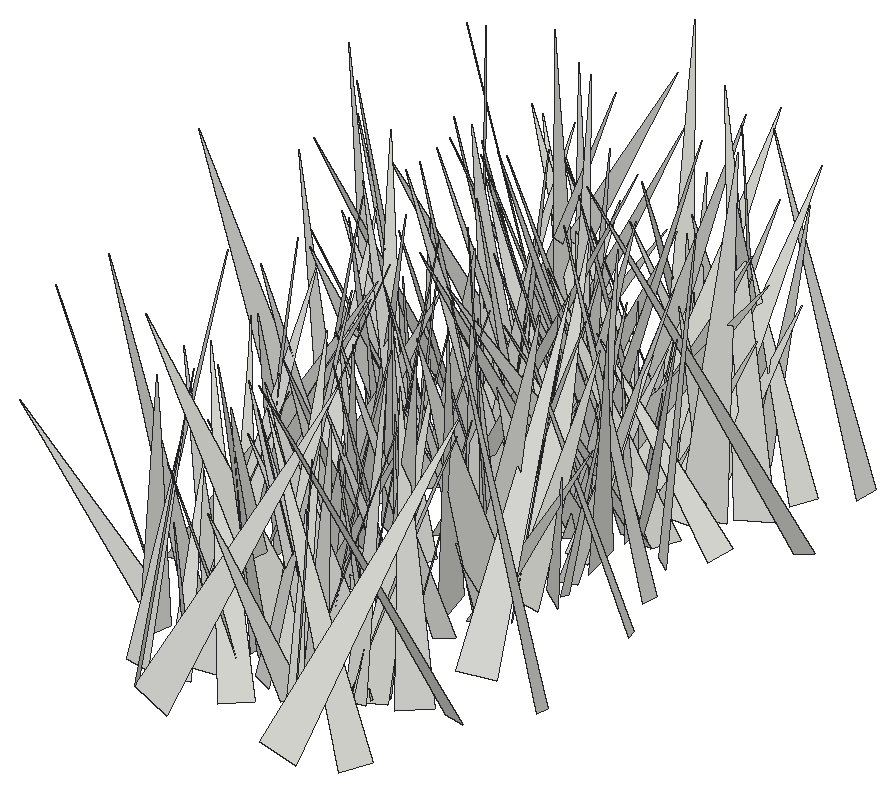
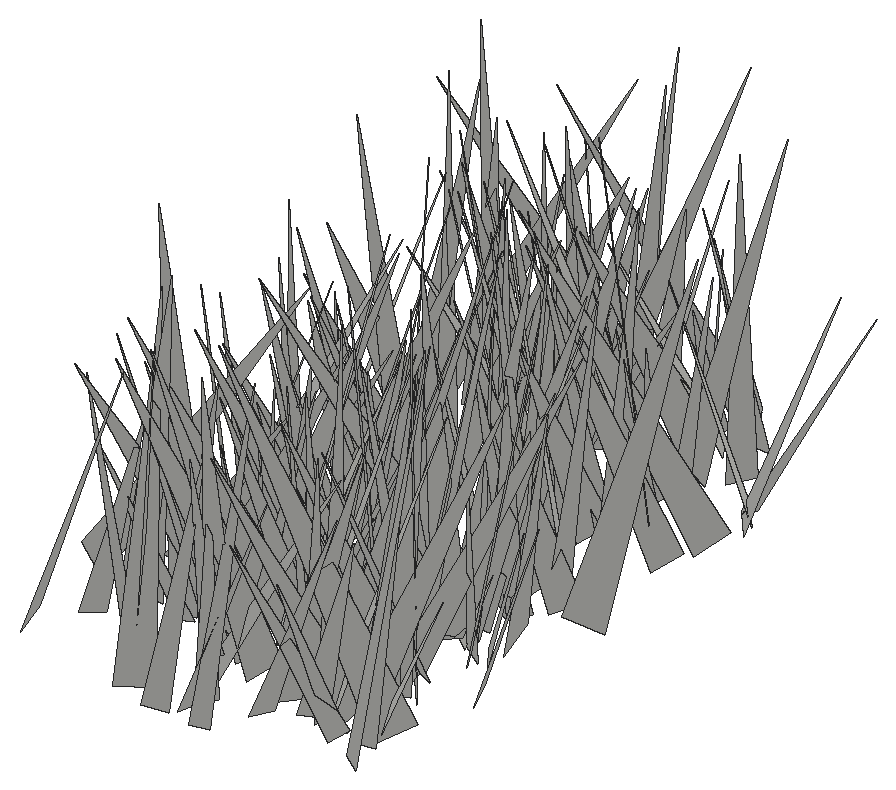
# SketchUp Ruby script. Lengths in inches.
U = 1.inch
M = Sketchup.active_model
def pt(a) = Geom::Point3d.new(a.map { |v| v * U })
def face(e, loops, mat)
  f = e.add_face(loops[0].map { |a| pt(a) })
  loops[1..].each { |l| e.add_face(l.map { |a| pt(a) }).erase! }
  f.material = f.back_material = mat if mat
  f
end
# faces: each face lists its corners as indices into pts; further lists are holes
def faces(e, pts, list, mat = nil) = list.each { |f| face(e, (f[0].is_a?(Array) ? f : [f]).map { |l| l.map { |i| pts[i] } }, mat) }
# xy, xz, yz: faces in a plane at the given z, y or x. An outline is a flat list of corners, or four numbers for a rectangle; further outlines are holes
def ring(l) = l.size == 4 ? [[l[0], l[1]], [l[2], l[1]], [l[2], l[3]], [l[0], l[3]]] : l.each_slice(2).to_a
def flat(e, list, mat, &to3) = list.each { |f| face(e, (f[0].is_a?(Array) ? f : [f]).map { |l| ring(l).map { |u, v| to3.(u, v) } }, mat) }
def xy(e, z, list, mat = nil) = flat(e, list, mat) { |x, y| [x, y, z] }
def xz(e, y, list, mat = nil) = flat(e, list, mat) { |x, z| [x, y, z] }
def yz(e, x, list, mat = nil) = flat(e, list, mat) { |y, z| [x, y, z] }
def lines(e, pts, list) = list.each { |a, b| e.add_line(pt(pts[a]), pt(pts[b])) }
# prism: a flat outline (further loops are holes) pulled along v
def prism(e, loops, v, mat = nil)
  f = face(e, loops, mat); d = Geom::Vector3d.new(v.map { |x| x * U })
  f.pushpull(f.normal.samedirection?(d) ? d.length : -d.length)
end
def box(e, o, s, mat = nil) = prism(e, [[o, [o[0] + s[0], o[1], o[2]], [o[0] + s[0], o[1] + s[1], o[2]], [o[0], o[1] + s[1], o[2]]]], [0, 0, s[2]], mat)
def at(x, y, z, deg = 0) = Geom::Transformation.translation(pt([x, y, z])) * Geom::Transformation.rotation(ORIGIN, Z_AXIS, deg.degrees)
def axes(o, x, y, z) = Geom::Transformation.new([*x, 0, *y, 0, *z, 0, *pt(o).to_a, 1])
def part(name) = M.definitions.add(name)
# library, detail: a bought-in or finely detailed component or shape, given as its bounding box
def library(name, o, s) = part(name).tap { |d| box(d.entities, o, s) }
def detail(e, o, s) = box(e.add_group.entities, o, s)
def put(e, d, t, mat = nil) = e.add_instance(d, t).tap { |i| i.material = mat if mat }
def group(e, t, mat = nil) = e.add_group.tap { |g| g.transformation = t; g.material = mat if mat }.entities
root = M.entities
c1 = part("fur_instance\#9")
p = [[0.8125,0,1.79],[0.67,-0.02,1.48],[0,-0.11,0],[0,0.11,0]]
faces(c1.entities,p,[[0,1,2,3]])
put(root,c1,axes([454.46,93.04,-21.66],[-5.41168,-1.42657,0.35166],[-1.45652,5.03228,-1.99993],[-0.1932,2.0214,5.22701]))
put(root,c1,axes([454.91,77.14,-21.66],[-4.61833,-3.74237,0.73758],[-3.79853,4.40694,-1.4242],[-0.34716,1.56584,5.77113]))
put(root,c1,axes([455.64,97.34,-21.66],[-4.45593,-2.02584,0.38216],[-1.95722,3.87117,-2.29973],[-0.64758,2.23951,4.32095]))
put(root,c1,axes([456,89.03,-21.66],[-7.80069,-0.47128,0.71432],[-0.70737,7.23754,-2.94972],[0.48165,2.99651,7.23686]))
put(root,c1,axes([454.72,86.68,-21.66],[1.74253,-7.39949,2.19817],[-7.33714,-2.28781,-1.88496],[-2.39807,1.62304,7.36449]))
put(root,c1,axes([455.25,76.27,-21.66],[-4.70731,-0.314,0.0439],[-0.28456,4.4722,1.47573],[0.13983,-1.46975,4.48103]))
put(root,c1,axes([455.95,90.67,-21.66],[-3.1769,-1.92196,0.83625],[-2.09296,2.82701,-1.45378],[-0.11299,1.67333,3.4166]))
put(root,c1,axes([454.96,99.93,-21.66],[-4.90749,-6.3294,1.61985],[-6.13533,5.16095,1.5783],[2.24565,0.26836,7.85199]))
put(root,c1,axes([455.21,76.35,-21.66],[4.3588,4.87451,1.02077],[4.50794,-4.43827,1.9448],[-2.11691,0.58556,6.24322]))
put(root,c1,axes([456.82,90.64,-21.86],[-6.58446,-3.61184,1.85584],[-3.84727,6.67992,-0.64953],[1.29924,1.4758,7.48189]))
put(root,c1,axes([458.16,92.25,-21.86],[-2.71774,-6.73125,0.47193],[-6.54696,2.5072,-1.9416],[-1.63394,1.15011,6.99472]))
put(root,c1,axes([457.14,85.11,-21.86],[-7.05246,-0.20222,1.59365],[-0.38202,7.18084,-0.77939],[1.56034,0.84409,7.01218]))
put(root,c1,axes([457.41,96,-21.66],[0.6668,-6.36542,0.43774],[-6.10772,-0.7641,-1.80742],[-1.84553,0.22889,6.13974]))
put(root,c1,axes([456.73,90.63,-21.86],[1.72426,4.07776,1.35625],[4.04188,-2.03524,0.98061],[-1.4597,-0.81871,4.31736]))
put(root,c1,axes([457.83,87.22,-21.86],[-1.06159,6.87885,0.56166],[6.76624,0.92524,1.45707],[-1.36093,-0.76575,6.80607]))
put(root,c1,axes([457.84,89.85,-21.86],[-4.26864,3.3889,1.68719],[3.78174,3.93314,1.66776],[0.17248,-2.36607,5.18889]))
put(root,c1,axes([455.38,98.63,-21.66],[-1.80775,-6.68688,0.47497],[-6.40102,1.86794,1.93536],[1.9917,-0.06601,6.65106]))
put(root,c1,axes([458.41,97.84,-21.86],[-3.43494,4.07646,0.13435],[4.04677,3.38429,0.77755],[-0.50915,-0.60283,5.27368]))
put(root,c1,axes([456.68,94,-21.86],[-5.7343,-4.84539,3.53032],[-5.45543,6.24306,-0.29262],[2.4858,2.5238,7.50162]))
put(root,c1,axes([457.64,97.98,-21.86],[-4.61159,-4.4726,0.38091],[-4.39573,4.61032,0.9157],[0.90928,-0.396,6.35865]))
put(root,c1,axes([457.61,90.15,-21.86],[-4.43936,-4.76816,0.23664],[-4.66276,4.39992,1.18262],[1.02469,-0.63608,6.40661]))
put(root,c1,axes([458.98,75.03,-21.86],[-2.69995,-7.06667,2.40673],[-7.39529,2.18224,-1.88876],[-1.01973,2.88442,7.32531]))
put(root,c1,axes([458.41,77.89,-21.66],[-4.8792,2.06982,0.10093],[1.96371,4.70056,-1.46614],[0.66196,1.31208,5.09325]))
put(root,c1,axes([455.8,80.76,-21.66],[1.53162,3.70831,1.75315],[4.01532,-0.97314,-1.44953],[0.83802,-2.1148,3.74116]))
put(root,c1,axes([458.52,76.28,-21.86],[-5.31115,0.249,1.00047],[0.14264,5.37711,-0.58108],[1.02108,0.54405,5.28514]))
put(root,c1,axes([457.35,89.66,-21.86],[-2.6203,-2.567,1.06702],[-2.53846,2.80716,0.51965],[1.13325,0.35259,3.63117]))
put(root,c1,axes([457.21,94.86,-21.86],[3.62749,-5.55241,1.8821],[-5.65778,-3.89547,-0.58748],[-1.5366,1.23544,6.60627]))
put(root,c1,axes([456.95,98.2,-21.86],[-0.81178,3.59213,0.55552],[3.51446,0.92094,-0.81938],[0.92765,-0.34562,3.5904]))
put(root,c1,axes([458.15,88.95,-21.86],[2.22572,-6.24997,0.53761],[-6.03536,-2.28904,-1.62473],[-1.71046,-0.05581,6.43243]))
put(root,c1,axes([457.19,87.79,-21.86],[-2.48382,-6.27006,1.58629],[-6.2632,2.75568,1.08533],[1.61318,1.04494,6.65621]))
put(root,c1,axes([457.4,92.89,-21.86],[2.05142,5.93925,0.09208],[5.90467,-2.04959,0.65232],[-0.64654,0.12643,6.2496]))
put(root,c1,axes([458.6875,81.05,-21.66],[-5.84983,3.65343,0.11485],[3.32744,5.4123,-2.68634],[1.51292,2.22277,6.35229]))
put(root,c1,axes([458.61,91.84,-21.86],[-5.55068,-3.03255,1.58004],[-3.06213,5.7489,0.27653],[1.52193,0.50669,6.31901]))
put(root,c1,axes([456.93,82.49,-21.86],[6.40589,-1.32849,1.4611],[-0.83624,-6.31798,-2.07823],[-1.78897,-1.80373,6.20333]))
put(root,c1,axes([456.87,94.24,-21.66],[6.5419,0.41912,1.71437],[-0.23349,-6.31856,2.43568],[-1.74935,2.41069,6.08602]))
put(root,c1,axes([457.17,74.36,-21.86],[5.79339,-2.08626,1.56673],[-1.97661,-6.00002,-0.68061],[-1.70297,-0.13319,6.11985]))
put(root,c1,axes([459.85,97.4375,-21.86],[-5.5849,2.54638,0.93821],[2.66389,5.55377,0.78405],[0.51763,-1.10771,6.08773]))
put(root,c1,axes([457.97,97.44,-21.86],[7.3985,0.06507,3.2704],[0.28828,-8.06925,-0.49163],[-3.25831,-0.56619,7.38244]))
put(root,c1,axes([455.27,81.11,-21.66],[6.30652,-2.10429,0.15189],[-2.07978,-6.12031,1.56194],[0.35446,1.52876,6.46224]))
put(root,c1,axes([460.03,98.8,-21.86],[-4.93751,1.50851,0.32737],[1.53378,4.91815,0.47027],[0.1741,-0.54591,5.14135]))
put(root,c1,axes([454.82,79.03,-21.66],[6.90826,-2.9112,0.5406],[-2.88435,-6.30625,2.89882],[0.66922,2.87186,6.91346]))
put(root,c1,axes([460.1,95.79,-21.66],[-6.71472,0.14595,1.05093],[-0.21339,6.41005,-2.25365],[1.03933,2.25902,6.32691]))
put(root,c1,axes([459.72,94.43,-21.86],[-4.78062,2.36193,1.12593],[2.54726,4.73726,0.87783],[0.59826,-1.2963,5.25951]))
put(root,c1,axes([458.15,72.125,-21.86],[0.58745,4.61701,1.14714],[4.75417,-0.52722,-0.31264],[0.17496,-1.17604,4.64372]))
put(root,c1,axes([457.01,87.52,-21.66],[1.41484,-4.55258,1.06253],[-4.54528,-1.07998,1.42506],[1.09333,1.40157,4.54939]))
put(root,c1,axes([455.04,97.26,-21.66],[6.5519,-4.81181,0.9912],[-4.80718,-5.93833,2.94799],[1.01342,2.94042,7.57563]))
put(root,c1,axes([458.58,80.55,-21.86],[6.51752,3.06728,2.32468],[2.5593,-6.86862,1.88745],[-2.87443,0.8392,6.95153]))
put(root,c1,axes([456.56,98.67,-21.66],[3.29977,-2.51906,0.3221],[-2.3698,-2.86445,1.87534],[0.91296,1.66948,3.70368]))
put(root,c1,axes([456,86.06,-21.66],[4.35594,-4.3452,0.48537],[-4.22774,-4.01128,2.03138],[1.11472,1.7662,5.80763]))
put(root,c1,axes([459.2,70.77,-21.66],[4.53649,3.63122,1.57008],[3.09166,-4.74451,2.04009],[-2.46831,0.73111,5.44092]))
put(root,c1,axes([457.15,96.9375,-21.66],[6.04009,-0.71684,0.90558],[-1.00409,-5.64184,2.23115],[-0.57074,2.3393,5.65849]))
put(root,c1,axes([457.88,85.74,-21.86],[6.8953,0.9557,1.85973],[1.13553,-7.09282,-0.56526],[-1.75571,-0.83402,6.93822]))
put(root,c1,axes([458.29,78.46,-21.86],[5.70767,4.90783,2.44546],[5.23724,-5.92496,-0.33273],[-1.62433,-1.85811,7.52021]))
put(root,c1,axes([460.06,72.18,-21.86],[-3.33951,2.40161,0.05247],[2.31618,3.24301,-1.02031],[0.63702,0.79874,3.98485]))
put(root,c1,axes([459.06,90.74,-21.86],[-3.15588,-6.30761,0.73503],[-6.08642,3.23856,1.65924],[1.81157,-0.10755,6.85511]))
put(root,c1,axes([458.95,87.48,-21.86],[4.97052,1.68586,2.30908],[2.28367,-5.12743,-1.17229],[-1.72012,-1.9358,5.11604]))
put(root,c1,axes([460.57,95.77,-21.86],[-4.85913,-4.7221,0.69622],[-4.68141,4.90862,0.61965],[0.93132,0.03646,6.74725]))
put(root,c1,axes([460.07,73.21,-21.86],[-6.65412,4.03174,0.74119],[3.28122,6.08544,-3.64454],[2.45722,2.79179,6.87384]))
put(root,c1,axes([460.8,81.57,-21.86],[-0.74223,-7.02206,1.66779],[-7.14663,0.48084,-1.156],[-1.00829,1.76103,6.96591]))
put(root,c1,axes([461.58,84.36,-21.86],[-7.31689,1.04904,1.18508],[0.99417,7.40794,-0.41938],[1.23147,0.25252,7.3798]))
put(root,c1,axes([461.99,91.53,-21.86],[-6.57116,-2.81105,0.67584],[-2.85659,6.57143,-0.44162],[0.44572,0.67315,7.13352]))
put(root,c1,axes([460.79,94.4,-21.86],[1.63726,6.8228,1.57078],[6.72877,-1.9791,1.58281],[-1.9343,-1.10957,6.83563]))
put(root,c1,axes([459.09,73.03,-21.66],[4.51704,3.2359,0.24642],[3.07452,-4.40221,1.45028],[-1.0388,1.04161,5.3639]))
put(root,c1,axes([458.53,93.53,-21.86],[5.45903,4.38742,2.52703],[5.0114,-5.21201,-1.77686],[-0.72192,-3.00365,6.77446]))
put(root,c1,axes([459.14,97.12,-21.86],[3.49606,4.56093,2.47636],[5.16488,-3.35013,-1.12142],[-0.50841,-2.67048,5.63622]))
put(root,c1,axes([459.72,73.15,-21.86],[3.15596,1.30372,1.61225],[1.82364,-3.14251,-1.02861],[-0.98659,-1.6383,3.25603]))
put(root,c1,axes([458.08,90.11,-21.86],[2.61473,-6.42495,0.46001],[-6.33227,-2.47287,1.45453],[1.18065,0.96609,6.78241]))
put(root,c1,axes([463.5,97.01,-21.86],[-4.82792,-3.85999,0.34861],[-3.62589,4.30173,-2.58417],[-1.36894,2.21934,5.6152]))
put(root,c1,axes([460.55,84.08,-21.86],[-3.5127,-1.06556,1.8883],[-1.54789,3.74984,-0.76344],[1.51826,1.35772,3.59049]))
put(root,c1,axes([459.48,90.96,-21.86],[1.6675,5.06938,1.93589],[5.41393,-1.41673,-0.95346],[0.36831,-2.12629,5.25072]))
put(root,c1,axes([462.75,72.17,-21.86],[-2.20757,6.36235,0.08993],[6.1827,2.12231,1.62203],[-1.50393,-0.61421,6.5362]))
put(root,c1,axes([463.15,76.28,-21.66],[-3.16767,-3.69393,0.44061],[-3.42422,2.66901,-2.24153],[-1.45395,1.76199,4.31912]))
put(root,c1,axes([461.22,81.45,-21.86],[-0.51846,-5.08764,2.15235],[-5.51728,0.36879,-0.45728],[-0.27624,2.18298,5.0935]))
put(root,c1,axes([462.54,88.77,-21.86],[-7.46338,-1.41905,1.28497],[-1.31215,7.55774,0.72509],[1.39396,-0.48353,7.56241]))
put(root,c1,axes([461.82,78.73,-21.66],[-4.35378,0.44066,1.23045],[0.84047,4.2213,1.46212],[1.0009,-1.62788,4.12453]))
put(root,c1,axes([463.04,76.02,-21.86],[-7.92224,1.63819,2.17065],[2.33717,7.51957,2.85498],[1.39032,-3.306,7.56932]))
put(root,c1,axes([458.48,77.75,-21.86],[7.55875,3.30018,0.58934],[3.3113,-7.57673,-0.04195],[-0.52327,-0.27436,8.24768]))
put(root,c1,axes([459.56,85.34,-21.86],[-1.15928,-6.64992,1.1524],[-6.36185,1.46707,2.06591],[2.25307,0.72087,6.42631]))
put(root,c1,axes([461.61,82.15,-21.86],[-1.29873,-6.18935,0.13887],[-6.18983,1.30082,0.08883],[0.11547,0.11765,6.32352]))
put(root,c1,axes([458.76,82.87,-21.66],[5.69332,3.04756,1.30745],[3.31373,-5.12843,-2.47574],[0.12746,-2.79687,5.96424]))
put(root,c1,axes([462.07,73.62,-21.86],[-3.79874,-3.55526,0.6962],[-3.51199,3.8615,0.55657],[0.88909,0.06302,5.17306]))
put(root,c1,axes([459.66,81.08,-21.66],[0.42063,-4.67833,0.35233],[-4.37367,-0.26302,1.72907],[1.69763,0.48155,4.36738]))
put(root,c1,axes([461.51,91.24,-21.66],[2.88186,3.44939,0.31018],[3.15851,-2.7832,1.60537],[-1.42067,0.8094,4.19835]))
put(root,c1,axes([462.43,100.3125,-21.86],[-4.26767,-0.91045,0.71231],[-0.70932,4.21373,1.13607],[0.91278,-0.98229,4.21323]))
put(root,c1,axes([462.72,78.72,-21.86],[-5.0365,1.95588,2.0654],[2.56555,4.93734,1.5806],[1.22852,-2.29236,5.16658]))
put(root,c1,axes([463.05,89.12,-21.86],[-6.09908,-2.25868,1.59557],[-2.41433,6.23322,-0.4051],[1.3485,0.94419,6.49124]))
put(root,c1,axes([460.95,101.3125,-21.66],[-1.84691,-6.18778,0.26193],[-5.9057,1.84189,1.87043],[1.86547,-0.29517,6.18071]))
put(root,c1,axes([462.92,91.46,-21.66],[-3.99864,-1.03805,0.42764],[-0.78188,3.71014,1.695],[0.80565,-1.55139,3.76744]))
put(root,c1,axes([460.89,76.36,-21.86],[6.56004,-2.8558,0.90961],[-2.50702,-6.42798,-2.10074],[-1.6425,-1.59457,6.83935]))
put(root,c1,axes([464.61,90.75,-21.66],[-5.23852,-3.39609,0.6769],[-3.443,4.97658,-1.67721],[-0.37061,1.77027,6.01352]))
put(root,c1,axes([463.03,85.49,-21.86],[0.97276,4.45119,0.9772],[4.35496,-1.20232,1.14148],[-1.3425,-0.67498,4.41093]))
put(root,c1,axes([460.31,81.86,-21.66],[-2.5118,-6.70095,1.69222],[-6.07027,2.9998,2.86854],[3.30427,0.41708,6.55616]))
put(root,c1,axes([459.875,95.25,-21.86],[5.28703,-2.12696,0.17156],[-2.11759,-5.17319,1.12251],[0.26309,1.10465,5.58719]))
put(root,c1,axes([461.25,88.28,-21.86],[4.90376,-2.85552,0.72078],[-2.73926,-4.93651,-0.92072],[-1.08166,-0.44414,5.59939]))
put(root,c1,axes([462.84,94.4,-21.66],[-6.10663,-5.12788,1.30944],[-4.81653,6.21333,1.86984],[2.19336,-0.63253,7.75176]))
put(root,c1,axes([461.76,89.29,-21.86],[2.82184,-3.33686,1.43593],[-3.57868,-2.86589,0.37288],[-0.62414,1.34588,4.35412]))
put(root,c1,axes([461.98,74.85,-21.86],[-3.5221,-6.63629,1.77015],[-6.5539,3.84233,1.36448],[2.0543,0.8804,7.38808]))
put(root,c1,axes([464.13,96.02,-21.66],[0.27633,8.1596,0.76138],[7.93766,-0.45592,2.00518],[-2.0377,-0.66947,7.91421]))
put(root,c1,axes([464.08,75.5625,-21.86],[-1.46223,5.38545,2.28823],[5.73287,0.84616,1.67196],[-1.17188,-2.58033,5.32407]))
put(root,c1,axes([463.5,95.35,-21.86],[-3.14093,-4.54056,1.19879],[-4.68857,3.11384,-0.49041],[0.26658,1.26749,5.49924]))
put(root,c1,axes([463.83,75.99,-21.86],[-4.56615,-2.82263,0.99228],[-2.92894,4.58662,-0.43101],[0.61084,0.89289,5.35081]))
put(root,c1,axes([462.22,99.31,-21.86],[3.44775,-2.42349,1.09947],[-2.43313,-3.5995,-0.30427],[-1.07797,0.37336,4.2033]))
put(root,c1,axes([462.83,74.91,-21.86],[-3.43213,5.64571,1.59286],[5.69776,3.64732,-0.65059],[1.39526,-1.00684,6.57497]))
put(root,c1,axes([462.75,73.68,-21.66],[4.10406,6.33899,0.98584],[6.11766,-4.2195,1.66374],[-1.93105,0.10466,7.36601]))
put(root,c1,axes([460.93,78.42,-21.86],[4.92318,-0.35306,0.35659],[-0.43613,-4.74982,1.31852],[-0.24819,1.34315,4.75646]))
put(root,c1,axes([462.81,81.47,-21.86],[-3.28751,-5.48957,1.02333],[-5.33666,3.43821,1.29963],[1.64396,0.18343,6.2653]))
put(root,c1,axes([461.02,86.39,-21.66],[7.74445,1.42991,0.81828],[1.0012,-7.20795,3.11989],[-1.30836,2.94814,7.231]))
put(root,c1,axes([460.21,70.35,-21.86],[0.84349,7.5995,0.98427],[7.14395,-0.42161,-2.86687],[2.77222,-1.22577,7.08837]))
put(root,c1,axes([464.17,89.71,-21.86],[-3.54918,2.04608,0.76374],[2.14815,3.53344,0.51649],[0.39398,-0.83357,4.06404]))
put(root,c1,axes([463.49,78.47,-21.66],[5.66789,4.81372,1.80284],[4.22946,-5.89252,2.43659],[-2.92126,0.80836,7.02566]))
put(root,c1,axes([464.25,80.35,-21.86],[-5.06877,-1.96642,0.89661],[-1.81084,5.11214,0.97466],[1.17965,-0.60192,5.34876]))
put(root,c1,axes([465.65,80.68,-21.86],[-0.2537,5.53184,2.90433],[5.7111,-0.97344,2.35297],[-2.53371,-2.74807,5.0129]))
put(root,c1,axes([463.29,100.96,-21.86],[1.69834,-4.62751,0.65795],[-4.61755,-1.76962,-0.52709],[-0.72459,0.43091,4.90106]))
put(root,c1,axes([462.875,92.79,-21.86],[-6.33754,-5.19611,0.8236],[-4.02771,5.62162,4.47406],[3.3846,-3.03975,6.86635]))
put(root,c1,axes([461.71,96.57,-21.66],[6.69974,-1.69034,1.74311],[-2.11177,-6.58131,1.73465],[-1.19837,2.1474,6.68841]))
put(root,c1,axes([463.42,88.61,-21.86],[3.60801,-2.69307,1.35493],[-2.4926,-3.85347,-1.02171],[-1.69571,-0.06573,4.3848]))
put(root,c1,axes([461.04,79.98,-21.66],[5.75664,2.23558,0.62086],[2.31995,-5.52205,-1.62697],[0.03364,-1.74108,5.95732]))
put(root,c1,axes([465.04,89.53,-21.66],[-0.88458,-7.33954,0.10795],[-7.20369,0.84713,-1.43254],[-1.40973,0.27658,7.25253]))
put(root,c1,axes([464.45,73.34,-21.66],[1.33499,-4.14938,1.03511],[-3.92508,-1.61935,-1.42916],[-1.69781,0.48101,4.1179]))
put(root,c1,axes([464.29,96.35,-21.66],[-5.1152,1.11044,1.16629],[0.73583,5.06638,-1.59654],[1.43244,1.36283,4.98492]))
put(root,c1,axes([462.15,78.35,-21.86],[4.41125,2.39111,1.26664],[2.67652,-4.21168,-1.37073],[-0.39751,-1.82353,4.82677]))
put(root,c1,axes([466.32,90.74,-21.86],[1.30343,6.50873,4.51627],[7.0846,-3.00591,2.28737],[-3.54523,-3.61388,6.23141]))
put(root,c1,axes([462.45,80.71,-21.86],[4.87544,3.99495,1.42226],[4.19795,-4.85335,-0.75795],[-0.59966,-1.4959,6.2574]))
put(root,c1,axes([463.58,93.07,-21.86],[3.51488,-3.51732,0.75482],[-3.443,-3.59499,-0.71937],[-1.04262,0.01399,4.9202]))
put(root,c1,axes([463.27,82.3125,-21.86],[3.50621,1.98379,0.78234],[2.0421,-3.55715,-0.13217],[-0.61424,-0.50223,4.02634]))
put(root,c1,axes([464.22,86.96,-21.86],[-2.71251,3.20119,0.88639],[3.03008,2.85354,-1.03292],[1.36084,0.02704,4.06674]))
put(root,c1,axes([466.11,82.48,-21.86],[-6.35383,-3.10693,1.06991],[-3.1587,6.41685,-0.12448],[0.9057,0.58302,7.07168]))
put(root,c1,axes([463.01,90.6,-21.86],[6.40804,-1.16691,1.44574],[-1.35043,-6.49108,0.74636],[-1.27601,1.00946,6.47052]))
put(root,c1,axes([465.3,85.375,-21.86],[-4.74866,-3.13825,0.27488],[-2.86364,4.50737,1.98925],[1.31291,-1.51952,5.33303]))
put(root,c1,axes([464.47,77.25,-21.86],[5.32818,4.49942,0.50618],[3.89144,-4.95023,3.04014],[-2.31467,2.03493,6.2763]))
put(root,c1,axes([465.04,84.11,-21.86],[-5.77727,-4.35757,2.82703],[-4.73437,6.15702,-0.18467],[2.13687,1.8601,7.23403]))
put(root,c1,axes([464.67,89.37,-21.86],[-6.96158,0.42843,3.50828],[-1.43896,6.73486,-3.67782],[3.22816,3.92599,5.92628]))
put(root,c1,axes([466.52,75.53,-21.86],[-4.28089,-1.18354,0.47624],[-1.27514,3.91753,-1.72642],[-0.03977,1.79046,4.09221]))
put(root,c1,axes([464.125,94.09,-21.86],[-4.61251,5.93847,1.25396],[5.3205,4.71401,-2.75381],[2.92064,0.79104,6.99694]))
put(root,c1,axes([465.36,86.34,-21.86],[-3.56616,5.34471,0.77163],[5.27091,3.64619,-0.89538],[1.17426,-0.13507,6.36253]))
put(root,c1,axes([466.98,90.6,-21.86],[-1.76635,-5.02439,0.02248],[-4.81779,1.68692,-1.51928],[-1.42615,0.52421,5.10454]))
put(root,c1,axes([464.79,79.51,-21.86],[-2.53313,-4.37285,1.78451],[-4.47538,2.86942,0.67851],[1.50904,1.16947,5.00781]))
put(root,c1,axes([464.41,89.77,-21.86],[4.7492,-0.22527,1.39473],[-0.44396,-4.88167,0.72329],[-1.34124,0.81823,4.6992]))
put(root,c1,axes([465.71,71.78,-21.86],[0.00503,4.167,0.7042],[4.17874,-0.11,0.62111],[-0.63075,-0.69557,4.12045]))
put(root,c1,axes([466.1,91.15,-21.86],[1.76698,3.75792,1.11012],[3.4505,-2.06932,1.51278],[-1.85698,-0.26926,3.86726]))
put(root,c1,axes([466.35,74.59,-21.66],[1.43264,6.02249,0.66756],[5.77311,-1.565,1.72927],[-1.84042,-0.22107,5.94411]))
put(root,c1,axes([465,73.83,-21.86],[5.47635,-0.94494,2.24683],[-1.1073,-5.8869,0.22307],[-2.17142,0.61884,5.55279]))
put(root,c1,axes([466.97,76.72,-21.86],[-6.75602,-0.97126,1.58692],[-1.43223,6.52998,-2.10085],[1.1876,2.34979,6.49412]))
put(root,c1,axes([465.03,72.76,-21.86],[4.34542,2.75412,2.00138],[2.98226,-4.64462,-0.0836],[-1.6422,-1.14703,5.14401]))
put(root,c1,axes([464.24,84.78,-21.86],[5.46763,0.70402,1.09334],[0.38726,-5.3924,1.5356],[-1.2414,1.41859,5.29457]))
put(root,c1,axes([464.96,92.97,-21.86],[3.22488,1.438,0.95498],[1.40641,-3.36208,0.31327],[-1.00092,-0.09099,3.51704]))
put(root,c1,axes([467.85,90.83,-21.66],[-2.55985,4.83206,1.74885],[4.89019,1.69025,2.4878],[-1.579,-2.59892,4.86955]))
put(root,c1,axes([462.65,96.0625,-21.66],[4.53332,-3.78068,0.06575],[-3.6354,-4.32956,1.69931],[1.04008,1.34544,5.65304]))
put(root,c1,axes([464.17,90.99,-21.86],[0.15011,3.96157,1.30257],[3.86973,0.35348,-1.52101],[1.55431,-1.26265,3.66102]))
put(root,c1,axes([469.15,71.14,-21.86],[-1.95645,6.57203,0.15793],[5.85701,1.66776,3.15567],[-2.98529,-1.03499,6.08778]))
put(root,c1,axes([466.38,98.1,-21.86],[-5.53367,-3.1899,2.46645],[-3.58117,5.81278,-0.51687],[1.85312,1.70777,6.3663]))
put(root,c1,axes([466.68,76.18,-21.86],[5.18637,5.57386,2.23152],[5.04396,-5.64447,2.37581],[-3.2567,0.13438,7.23339]))
put(root,c1,axes([463.77,96.65,-21.66],[3.63408,5.21962,1.38175],[5.32326,-3.18476,-1.96987],[0.90365,-2.23003,6.04736]))
put(root,c1,axes([465.68,89.51,-21.86],[-2.04646,-5.42862,2.85461],[-5.95901,2.47232,0.42963],[1.45222,2.49488,5.78561]))
put(root,c1,axes([462.32,93.58,-21.86],[4.62991,-4.98565,0.093],[-4.3743,-3.99984,3.34189],[2.39393,2.33366,5.92659]))
put(root,c1,axes([464.78,82.1,-21.66],[7.73874,0.04549,1.82687],[0.5794,-7.60007,-2.26513],[-1.73315,-2.33761,7.39995]))
put(root,c1,axes([465.82,83.38,-21.66],[6.63906,-4.24471,1.17982],[-3.75911,-6.57064,-2.48644],[-2.29753,-1.51516,7.47745]))
put(root,c1,axes([464.9,100.13,-21.86],[5.93446,-4.51627,0.11992],[-4.41947,-5.84426,-1.3935],[-0.93776,-1.03771,7.32616]))
put(root,c1,axes([465.73,88.29,-21.86],[-0.65991,4.20046,0.70673],[4.09857,0.8209,-1.05196],[1.15975,-0.51096,4.1198]))
put(root,c1,axes([466.67,83.33,-21.86],[3.7445,3.22853,1.26331],[2.91821,-3.9391,1.41711],[-1.87174,0.31742,4.73672]))
put(root,c1,axes([466.3,90.75,-21.86],[-3.40135,-0.48301,1.73948],[-0.24917,3.80046,0.56808],[1.78802,-0.38922,3.38818]))
put(root,c1,axes([466.54,75.17,-21.86],[-4.85985,3.92503,1.53679],[3.59209,5.08366,-1.6245],[2.20555,0.36911,6.032]))
put(root,c1,axes([466.81,94.94,-21.86],[2.46831,-3.73303,1.12427],[-3.72872,-2.64901,-0.60947],[-1.13849,0.58247,4.43358]))
put(root,c1,axes([469.94,75.86,-21.66],[-3.80092,-6.72254,0.0507],[-6.48684,3.65215,-2.05545],[-1.76524,1.05421,7.4441]))
put(root,c1,axes([466.62,86.66,-21.86],[5.42,0.95377,1.93695],[-0.10115,-5.11614,2.80228],[-2.15667,2.63692,4.73638]))
put(root,c1,axes([464.75,78.92,-21.66],[-0.13317,-8.12567,1.45261],[-7.87911,0.55826,2.40046],[2.46092,1.34765,7.76415]))
put(root,c1,axes([465.51,75.09,-21.86],[4.56753,3.50086,0.36537],[3.49009,-4.58212,0.27435],[-0.45689,-0.00383,5.74831]))
put(root,c1,axes([469.95,87.29,-21.66],[-6.83624,-2.0461,0.45627],[-2.08301,6.45462,-2.26447],[-0.23611,2.29788,6.76704]))
put(root,c1,axes([469.67,91.76,-21.86],[-3.75948,2.94392,0.27379],[2.73653,3.29698,2.12525],[-1.1194,-1.82718,4.27594]))
put(root,c1,axes([467.33,85.59,-21.66],[3.33394,1.47543,1.26624],[0.9738,-3.44268,1.44745],[-1.68284,0.93087,3.34618]))
put(root,c1,axes([465.17,83.64,-21.66],[0.9927,-7.18833,2.00129],[-7.23058,-0.4281,2.04891],[1.84279,2.19257,6.96128]))
put(root,c1,axes([469.06,94.52,-21.86],[-1.50956,7.97784,1.83345],[8.07703,1.14872,1.65178],[-1.3301,-2.07864,7.94961]))
put(root,c1,axes([466.24,98.51,-21.86],[-1.49797,-4.88201,2.75569],[-5.27998,2.18724,1.00478],[1.88406,2.24805,5.00683]))
put(root,c1,axes([471.05,84.82,-21.66],[-6.43148,-3.95381,0.27263],[-3.76371,5.93049,-2.78112],[-1.24153,2.50351,7.01869]))
put(root,c1,axes([465.81,93.15,-21.86],[3.57113,-2.0967,0.79041],[-2.23153,-3.1932,1.61171],[0.20288,1.78359,3.81464]))
put(root,c1,axes([468.15,75.82,-21.86],[-4.07853,4.6775,2.02917],[4.97181,4.22458,0.25488],[1.13033,-1.70436,6.20068]))
put(root,c1,axes([467.12,92.49,-21.66],[-4.67484,5.38464,0.57126],[4.73589,4.43174,-3.01759],[2.62527,1.59378,6.46085]))
put(root,c1,axes([468.3,79.22,-21.86],[-5.16112,5.15909,0.10388],[4.87926,4.92701,-2.27629],[1.67923,1.54029,6.93338]))
put(root,c1,axes([466.51,95.13,-21.86],[0.4921,4.23207,0.57816],[4.10963,-0.31046,-1.22532],[1.16432,-0.69285,4.08059]))
put(root,c1,axes([471.96,93.76,-21.86],[-3.41379,-7.32141,0.63154],[-6.65452,2.7845,-3.69049],[-3.11756,2.07349,7.18591]))
put(root,c1,axes([466.52,84.16,-21.66],[-0.20342,5.45726,1.92359],[5.57072,0.70526,-1.41173],[1.56492,-1.80117,5.27542]))
put(root,c1,axes([468.4,89.95,-21.86],[3.82909,4.88275,1.88302],[4.81565,-4.20088,1.10051],[-2.04855,-0.74856,6.10673]))
put(root,c1,axes([466.6,88.6,-21.86],[6.47505,-0.26988,1.20187],[0.07267,-6.33614,-1.81428],[-1.22965,-1.79557,6.22153]))
put(root,c1,axes([466.07,82.13,-21.66],[4.34648,-1.55951,0.20323],[-1.53377,-4.07129,1.56122],[0.34774,1.53551,4.34586]))
put(root,c1,axes([466.85,90.71,-21.86],[5.2345,0.58731,0.96902],[0.7581,-5.21929,-0.93179],[-0.84215,-1.04786,5.18428]))
put(root,c1,axes([466.93,85.36,-21.86],[-1.05562,-3.90874,0.84941],[-3.49411,1.32871,1.77194],[1.94702,0.26528,3.64044]))
put(root,c1,axes([471.02,98.58,-21.86],[-7.05105,-1.29004,0.36767],[-1.33665,6.92247,-1.34515],[0.11284,1.38992,7.04075]))
put(root,c1,axes([467.53,93.4,-21.86],[-3.47226,6.33449,3.63746],[6.89094,4.17667,-0.69553],[2.42317,-2.80055,7.19017]))
put(root,c1,axes([469.56,96.73,-21.86],[-4.02277,2.62654,1.01722],[2.78428,3.97624,0.74391],[0.42575,-1.18612,4.74637]))
put(root,c1,axes([466.51,69.88,-21.66],[-0.73588,7.38124,0.25307],[6.98236,0.77818,-2.39362],[2.40696,-0.00075,7.02103]))
put(root,c1,axes([471.8125,78.66,-21.86],[-7.1733,-2.93015,0.73361],[-2.97558,6.52972,-3.01478],[-0.51951,3.05896,7.13815]))
